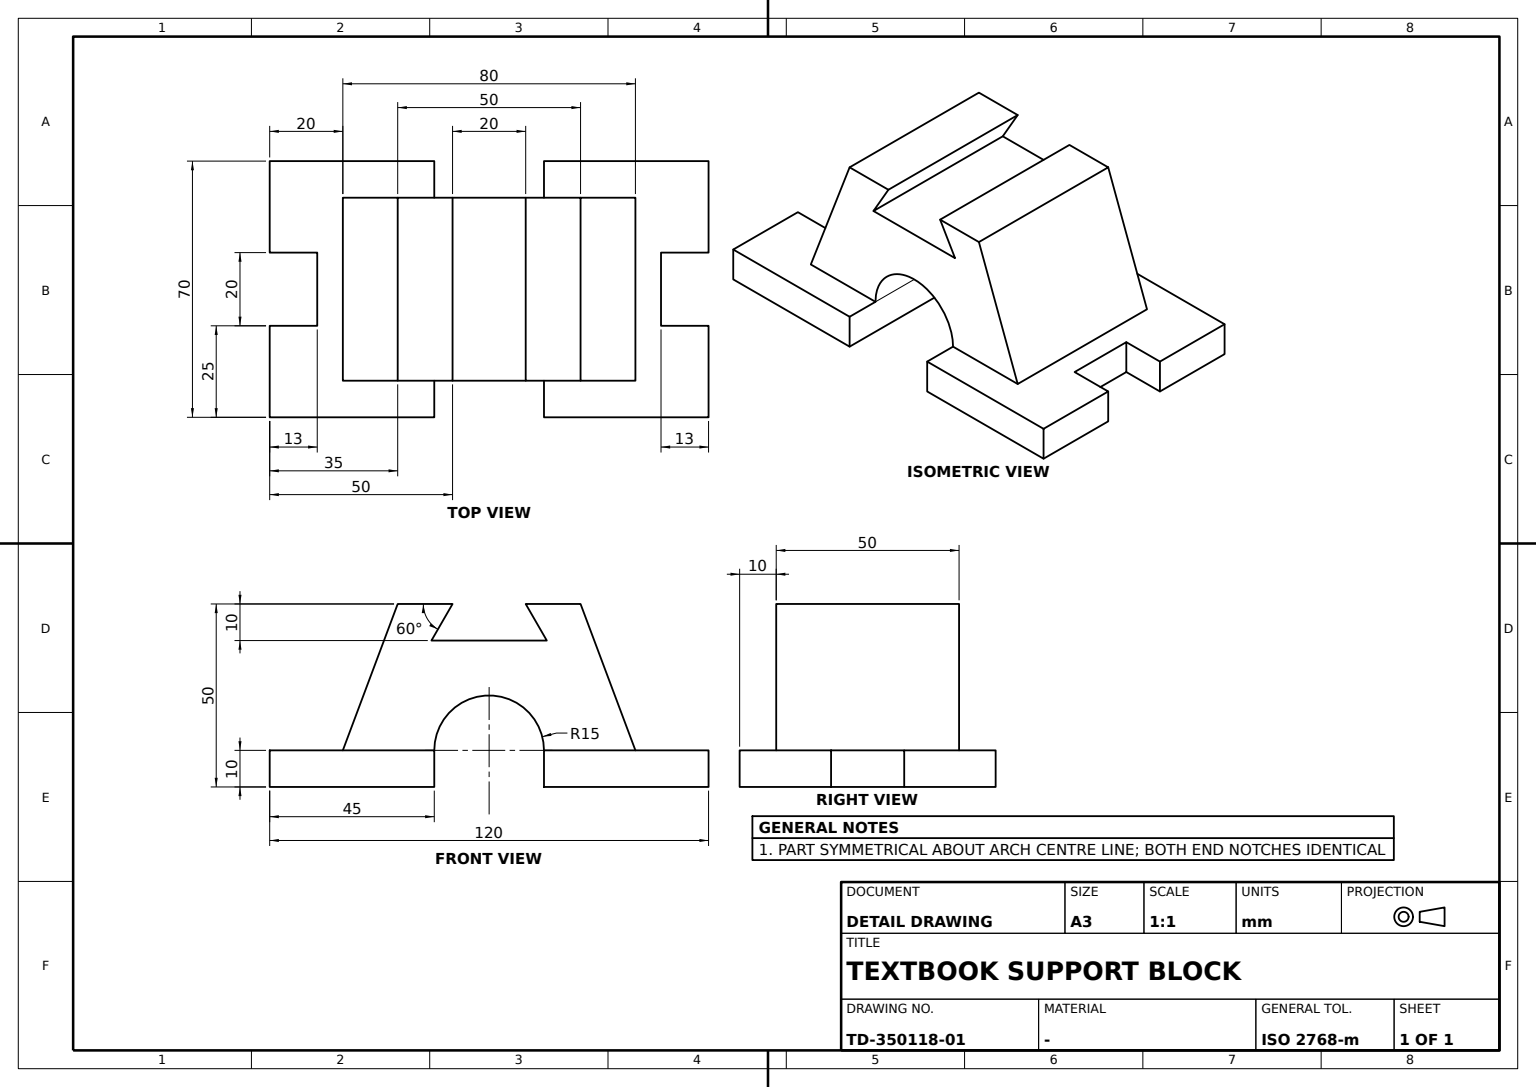
ISO-10303-21;
HEADER;
FILE_DESCRIPTION((''),'2;1');
FILE_NAME('','',(''),(''),'','','');
FILE_SCHEMA(('AUTOMOTIVE_DESIGN'));
ENDSEC;
DATA;
#1=APPLICATION_CONTEXT('');
#2=PRODUCT_CONTEXT('',#1,'mechanical');
#3=PRODUCT('','','',(#2));
#4=PRODUCT_DEFINITION_FORMATION('','',#3);
#5=PRODUCT_DEFINITION_CONTEXT('',#1,'design');
#6=PRODUCT_DEFINITION('','',#4,#5);
#7=PRODUCT_DEFINITION_SHAPE('','',#6);
#8=(LENGTH_UNIT()NAMED_UNIT(*)SI_UNIT(.MILLI.,.METRE.));
#9=(NAMED_UNIT(*)PLANE_ANGLE_UNIT()SI_UNIT($,.RADIAN.));
#10=(NAMED_UNIT(*)SI_UNIT($,.STERADIAN.)SOLID_ANGLE_UNIT());
#11=UNCERTAINTY_MEASURE_WITH_UNIT(LENGTH_MEASURE(1.E-05),#8,'distance_accuracy_value','');
#12=(GEOMETRIC_REPRESENTATION_CONTEXT(3)GLOBAL_UNCERTAINTY_ASSIGNED_CONTEXT((#11))GLOBAL_UNIT_ASSIGNED_CONTEXT((#8,#9,#10))REPRESENTATION_CONTEXT('',''));
#13=CARTESIAN_POINT('',(40.,25.,10.));
#14=VERTEX_POINT('',#13);
#15=CARTESIAN_POINT('',(15.,25.,10.));
#16=VERTEX_POINT('',#15);
#17=CARTESIAN_POINT('',(27.5,25.,10.));
#18=DIRECTION('',(-1.,0.,0.));
#19=VECTOR('',#18,1000.);
#20=LINE('',#17,#19);
#21=EDGE_CURVE('',#14,#16,#20,.T.);
#22=ORIENTED_EDGE('',*,*,#21,.F.);
#23=CARTESIAN_POINT('',(40.,-25.,10.));
#24=VERTEX_POINT('',#23);
#25=CARTESIAN_POINT('',(40.,0.,10.));
#26=DIRECTION('',(0.,1.,0.));
#27=VECTOR('',#26,1000.);
#28=LINE('',#25,#27);
#29=EDGE_CURVE('',#24,#14,#28,.T.);
#30=ORIENTED_EDGE('',*,*,#29,.F.);
#31=CARTESIAN_POINT('',(15.,-25.,10.));
#32=VERTEX_POINT('',#31);
#33=CARTESIAN_POINT('',(27.5,-25.,10.));
#34=LINE('',#33,#19);
#35=EDGE_CURVE('',#24,#32,#34,.T.);
#36=ORIENTED_EDGE('',*,*,#35,.T.);
#37=CARTESIAN_POINT('',(15.,-35.,10.));
#38=VERTEX_POINT('',#37);
#39=CARTESIAN_POINT('',(15.,-30.,10.));
#40=LINE('',#39,#27);
#41=EDGE_CURVE('',#38,#32,#40,.T.);
#42=ORIENTED_EDGE('',*,*,#41,.F.);
#43=CARTESIAN_POINT('',(60.,-35.,10.));
#44=VERTEX_POINT('',#43);
#45=CARTESIAN_POINT('',(37.5,-35.,10.));
#46=DIRECTION('',(1.,0.,0.));
#47=VECTOR('',#46,1000.);
#48=LINE('',#45,#47);
#49=EDGE_CURVE('',#38,#44,#48,.T.);
#50=ORIENTED_EDGE('',*,*,#49,.T.);
#51=CARTESIAN_POINT('',(60.,-10.,10.));
#52=VERTEX_POINT('',#51);
#53=CARTESIAN_POINT('',(60.,-22.5,10.));
#54=LINE('',#53,#27);
#55=EDGE_CURVE('',#44,#52,#54,.T.);
#56=ORIENTED_EDGE('',*,*,#55,.T.);
#57=CARTESIAN_POINT('',(47.,-10.,10.));
#58=VERTEX_POINT('',#57);
#59=CARTESIAN_POINT('',(53.5,-10.,10.));
#60=LINE('',#59,#47);
#61=EDGE_CURVE('',#58,#52,#60,.T.);
#62=ORIENTED_EDGE('',*,*,#61,.F.);
#63=CARTESIAN_POINT('',(47.,10.,10.));
#64=VERTEX_POINT('',#63);
#65=CARTESIAN_POINT('',(47.,0.,10.));
#66=DIRECTION('',(0.,-1.,0.));
#67=VECTOR('',#66,1000.);
#68=LINE('',#65,#67);
#69=EDGE_CURVE('',#64,#58,#68,.T.);
#70=ORIENTED_EDGE('',*,*,#69,.F.);
#71=CARTESIAN_POINT('',(60.,10.,10.));
#72=VERTEX_POINT('',#71);
#73=CARTESIAN_POINT('',(53.5,10.,10.));
#74=LINE('',#73,#19);
#75=EDGE_CURVE('',#72,#64,#74,.T.);
#76=ORIENTED_EDGE('',*,*,#75,.F.);
#77=CARTESIAN_POINT('',(60.,35.,10.));
#78=VERTEX_POINT('',#77);
#79=CARTESIAN_POINT('',(60.,22.5,10.));
#80=LINE('',#79,#27);
#81=EDGE_CURVE('',#72,#78,#80,.T.);
#82=ORIENTED_EDGE('',*,*,#81,.T.);
#83=CARTESIAN_POINT('',(15.,35.,10.));
#84=VERTEX_POINT('',#83);
#85=CARTESIAN_POINT('',(37.5,35.,10.));
#86=LINE('',#85,#19);
#87=EDGE_CURVE('',#78,#84,#86,.T.);
#88=ORIENTED_EDGE('',*,*,#87,.T.);
#89=CARTESIAN_POINT('',(15.,30.,10.));
#90=LINE('',#89,#27);
#91=EDGE_CURVE('',#16,#84,#90,.T.);
#92=ORIENTED_EDGE('',*,*,#91,.F.);
#93=EDGE_LOOP('',(#22,#30,#36,#42,#50,#56,#62,#70,#76,#82,#88,#92));
#94=FACE_OUTER_BOUND('',#93,.T.);
#95=CARTESIAN_POINT('',(0.,0.,10.));
#96=DIRECTION('',(0.,0.,1.));
#97=AXIS2_PLACEMENT_3D('',#95,#96,#46);
#98=PLANE('',#97);
#99=ADVANCED_FACE('',(#94),#98,.T.);
#100=CARTESIAN_POINT('',(25.,25.,50.));
#101=VERTEX_POINT('',#100);
#102=CARTESIAN_POINT('',(32.5,25.,30.));
#103=DIRECTION('',(0.351123442,0.,-0.936329178));
#104=VECTOR('',#103,1000.);
#105=LINE('',#102,#104);
#106=EDGE_CURVE('',#101,#14,#105,.T.);
#107=ORIENTED_EDGE('',*,*,#106,.T.);
#108=ORIENTED_EDGE('',*,*,#21,.T.);
#109=CARTESIAN_POINT('',(-15.,25.,10.));
#110=VERTEX_POINT('',#109);
#111=CARTESIAN_POINT('',(0.,25.,10.));
#112=AXIS2_PLACEMENT_3D('',#111,#26,#18);
#113=CIRCLE('',#112,15.);
#114=EDGE_CURVE('',#110,#16,#113,.T.);
#115=ORIENTED_EDGE('',*,*,#114,.F.);
#116=CARTESIAN_POINT('',(-40.,25.,10.));
#117=VERTEX_POINT('',#116);
#118=CARTESIAN_POINT('',(-27.5,25.,10.));
#119=LINE('',#118,#19);
#120=EDGE_CURVE('',#110,#117,#119,.T.);
#121=ORIENTED_EDGE('',*,*,#120,.T.);
#122=CARTESIAN_POINT('',(-25.,25.,50.));
#123=VERTEX_POINT('',#122);
#124=CARTESIAN_POINT('',(-32.5,25.,30.));
#125=DIRECTION('',(0.351123442,0.,0.936329178));
#126=VECTOR('',#125,1000.);
#127=LINE('',#124,#126);
#128=EDGE_CURVE('',#117,#123,#127,.T.);
#129=ORIENTED_EDGE('',*,*,#128,.T.);
#130=CARTESIAN_POINT('',(-10.,25.,50.));
#131=VERTEX_POINT('',#130);
#132=CARTESIAN_POINT('',(-17.5,25.,50.));
#133=LINE('',#132,#47);
#134=EDGE_CURVE('',#123,#131,#133,.T.);
#135=ORIENTED_EDGE('',*,*,#134,.T.);
#136=CARTESIAN_POINT('',(-15.773503,25.,40.));
#137=VERTEX_POINT('',#136);
#138=CARTESIAN_POINT('',(-12.886751,25.,45.));
#139=DIRECTION('',(-0.5,0.,-0.866025404));
#140=VECTOR('',#139,1000.);
#141=LINE('',#138,#140);
#142=EDGE_CURVE('',#131,#137,#141,.T.);
#143=ORIENTED_EDGE('',*,*,#142,.T.);
#144=CARTESIAN_POINT('',(15.773503,25.,40.));
#145=VERTEX_POINT('',#144);
#146=CARTESIAN_POINT('',(0.,25.,40.));
#147=LINE('',#146,#47);
#148=EDGE_CURVE('',#137,#145,#147,.T.);
#149=ORIENTED_EDGE('',*,*,#148,.T.);
#150=CARTESIAN_POINT('',(10.,25.,50.));
#151=VERTEX_POINT('',#150);
#152=CARTESIAN_POINT('',(12.886751,25.,45.));
#153=DIRECTION('',(0.5,0.,-0.866025404));
#154=VECTOR('',#153,1000.);
#155=LINE('',#152,#154);
#156=EDGE_CURVE('',#151,#145,#155,.T.);
#157=ORIENTED_EDGE('',*,*,#156,.F.);
#158=CARTESIAN_POINT('',(17.5,25.,50.));
#159=LINE('',#158,#47);
#160=EDGE_CURVE('',#151,#101,#159,.T.);
#161=ORIENTED_EDGE('',*,*,#160,.T.);
#162=EDGE_LOOP('',(#107,#108,#115,#121,#129,#135,#143,#149,#157,#161));
#163=FACE_OUTER_BOUND('',#162,.T.);
#164=CARTESIAN_POINT('',(0.,25.,0.));
#165=AXIS2_PLACEMENT_3D('',#164,#26,#18);
#166=PLANE('',#165);
#167=ADVANCED_FACE('',(#163),#166,.T.);
#168=CARTESIAN_POINT('',(-60.,-10.,0.));
#169=VERTEX_POINT('',#168);
#170=CARTESIAN_POINT('',(-47.,-10.,0.));
#171=VERTEX_POINT('',#170);
#172=CARTESIAN_POINT('',(-53.5,-10.,0.));
#173=LINE('',#172,#47);
#174=EDGE_CURVE('',#169,#171,#173,.T.);
#175=ORIENTED_EDGE('',*,*,#174,.T.);
#176=CARTESIAN_POINT('',(-47.,10.,0.));
#177=VERTEX_POINT('',#176);
#178=CARTESIAN_POINT('',(-47.,0.,0.));
#179=LINE('',#178,#27);
#180=EDGE_CURVE('',#171,#177,#179,.T.);
#181=ORIENTED_EDGE('',*,*,#180,.T.);
#182=CARTESIAN_POINT('',(-60.,10.,0.));
#183=VERTEX_POINT('',#182);
#184=CARTESIAN_POINT('',(-53.5,10.,0.));
#185=LINE('',#184,#47);
#186=EDGE_CURVE('',#183,#177,#185,.T.);
#187=ORIENTED_EDGE('',*,*,#186,.F.);
#188=CARTESIAN_POINT('',(-60.,35.,0.));
#189=VERTEX_POINT('',#188);
#190=CARTESIAN_POINT('',(-60.,22.5,0.));
#191=LINE('',#190,#67);
#192=EDGE_CURVE('',#189,#183,#191,.T.);
#193=ORIENTED_EDGE('',*,*,#192,.F.);
#194=CARTESIAN_POINT('',(-15.,35.,0.));
#195=VERTEX_POINT('',#194);
#196=CARTESIAN_POINT('',(-37.5,35.,0.));
#197=LINE('',#196,#19);
#198=EDGE_CURVE('',#195,#189,#197,.T.);
#199=ORIENTED_EDGE('',*,*,#198,.F.);
#200=CARTESIAN_POINT('',(-15.,-35.,0.));
#201=VERTEX_POINT('',#200);
#202=CARTESIAN_POINT('',(-15.,0.,0.));
#203=LINE('',#202,#27);
#204=EDGE_CURVE('',#201,#195,#203,.T.);
#205=ORIENTED_EDGE('',*,*,#204,.F.);
#206=CARTESIAN_POINT('',(-60.,-35.,0.));
#207=VERTEX_POINT('',#206);
#208=CARTESIAN_POINT('',(-37.5,-35.,0.));
#209=LINE('',#208,#47);
#210=EDGE_CURVE('',#207,#201,#209,.T.);
#211=ORIENTED_EDGE('',*,*,#210,.F.);
#212=CARTESIAN_POINT('',(-60.,-22.5,0.));
#213=LINE('',#212,#67);
#214=EDGE_CURVE('',#169,#207,#213,.T.);
#215=ORIENTED_EDGE('',*,*,#214,.F.);
#216=EDGE_LOOP('',(#175,#181,#187,#193,#199,#205,#211,#215));
#217=FACE_OUTER_BOUND('',#216,.T.);
#218=CARTESIAN_POINT('',(0.,0.,0.));
#219=AXIS2_PLACEMENT_3D('',#218,#96,#46);
#220=PLANE('',#219);
#221=ADVANCED_FACE('',(#217),#220,.F.);
#222=CARTESIAN_POINT('',(47.,10.,0.));
#223=VERTEX_POINT('',#222);
#224=CARTESIAN_POINT('',(47.,10.,5.));
#225=DIRECTION('',(0.,0.,-1.));
#226=VECTOR('',#225,1000.);
#227=LINE('',#224,#226);
#228=EDGE_CURVE('',#64,#223,#227,.T.);
#229=ORIENTED_EDGE('',*,*,#228,.F.);
#230=ORIENTED_EDGE('',*,*,#69,.T.);
#231=CARTESIAN_POINT('',(47.,-10.,0.));
#232=VERTEX_POINT('',#231);
#233=CARTESIAN_POINT('',(47.,-10.,5.));
#234=LINE('',#233,#226);
#235=EDGE_CURVE('',#58,#232,#234,.T.);
#236=ORIENTED_EDGE('',*,*,#235,.T.);
#237=CARTESIAN_POINT('',(47.,0.,0.));
#238=LINE('',#237,#27);
#239=EDGE_CURVE('',#232,#223,#238,.T.);
#240=ORIENTED_EDGE('',*,*,#239,.T.);
#241=EDGE_LOOP('',(#229,#230,#236,#240));
#242=FACE_OUTER_BOUND('',#241,.T.);
#243=AXIS2_PLACEMENT_3D('',#57,#18,#26);
#244=PLANE('',#243);
#245=ADVANCED_FACE('',(#242),#244,.F.);
#246=CARTESIAN_POINT('',(60.,-35.,0.));
#247=VERTEX_POINT('',#246);
#248=CARTESIAN_POINT('',(60.,-35.,5.));
#249=VECTOR('',#96,1000.);
#250=LINE('',#248,#249);
#251=EDGE_CURVE('',#247,#44,#250,.T.);
#252=ORIENTED_EDGE('',*,*,#251,.T.);
#253=ORIENTED_EDGE('',*,*,#49,.F.);
#254=CARTESIAN_POINT('',(15.,-35.,0.));
#255=VERTEX_POINT('',#254);
#256=CARTESIAN_POINT('',(15.,-35.,5.));
#257=LINE('',#256,#249);
#258=EDGE_CURVE('',#255,#38,#257,.T.);
#259=ORIENTED_EDGE('',*,*,#258,.F.);
#260=CARTESIAN_POINT('',(37.5,-35.,0.));
#261=LINE('',#260,#47);
#262=EDGE_CURVE('',#255,#247,#261,.T.);
#263=ORIENTED_EDGE('',*,*,#262,.T.);
#264=EDGE_LOOP('',(#252,#253,#259,#263));
#265=FACE_OUTER_BOUND('',#264,.T.);
#266=AXIS2_PLACEMENT_3D('',#246,#26,#18);
#267=PLANE('',#266);
#268=ADVANCED_FACE('',(#265),#267,.F.);
#269=CARTESIAN_POINT('',(60.,10.,0.));
#270=VERTEX_POINT('',#269);
#271=CARTESIAN_POINT('',(60.,10.,5.));
#272=LINE('',#271,#226);
#273=EDGE_CURVE('',#72,#270,#272,.T.);
#274=ORIENTED_EDGE('',*,*,#273,.F.);
#275=ORIENTED_EDGE('',*,*,#75,.T.);
#276=ORIENTED_EDGE('',*,*,#228,.T.);
#277=CARTESIAN_POINT('',(53.5,10.,0.));
#278=LINE('',#277,#19);
#279=EDGE_CURVE('',#270,#223,#278,.T.);
#280=ORIENTED_EDGE('',*,*,#279,.F.);
#281=EDGE_LOOP('',(#274,#275,#276,#280));
#282=FACE_OUTER_BOUND('',#281,.T.);
#283=AXIS2_PLACEMENT_3D('',#63,#26,#46);
#284=PLANE('',#283);
#285=ADVANCED_FACE('',(#282),#284,.F.);
#286=CARTESIAN_POINT('',(-15.,-35.,10.));
#287=VERTEX_POINT('',#286);
#288=CARTESIAN_POINT('',(-15.,-35.,5.));
#289=LINE('',#288,#226);
#290=EDGE_CURVE('',#287,#201,#289,.T.);
#291=ORIENTED_EDGE('',*,*,#290,.F.);
#292=CARTESIAN_POINT('',(-60.,-35.,10.));
#293=VERTEX_POINT('',#292);
#294=CARTESIAN_POINT('',(-37.5,-35.,10.));
#295=LINE('',#294,#47);
#296=EDGE_CURVE('',#293,#287,#295,.T.);
#297=ORIENTED_EDGE('',*,*,#296,.F.);
#298=CARTESIAN_POINT('',(-60.,-35.,5.));
#299=LINE('',#298,#249);
#300=EDGE_CURVE('',#207,#293,#299,.T.);
#301=ORIENTED_EDGE('',*,*,#300,.F.);
#302=ORIENTED_EDGE('',*,*,#210,.T.);
#303=EDGE_LOOP('',(#291,#297,#301,#302));
#304=FACE_OUTER_BOUND('',#303,.T.);
#305=ADVANCED_FACE('',(#304),#267,.F.);
#306=CARTESIAN_POINT('',(-40.,-25.,10.));
#307=VERTEX_POINT('',#306);
#308=CARTESIAN_POINT('',(-40.,0.,10.));
#309=LINE('',#308,#27);
#310=EDGE_CURVE('',#307,#117,#309,.T.);
#311=ORIENTED_EDGE('',*,*,#310,.F.);
#312=CARTESIAN_POINT('',(-25.,-25.,50.));
#313=VERTEX_POINT('',#312);
#314=CARTESIAN_POINT('',(-32.5,-25.,30.));
#315=LINE('',#314,#126);
#316=EDGE_CURVE('',#307,#313,#315,.T.);
#317=ORIENTED_EDGE('',*,*,#316,.T.);
#318=CARTESIAN_POINT('',(-25.,0.,50.));
#319=LINE('',#318,#27);
#320=EDGE_CURVE('',#313,#123,#319,.T.);
#321=ORIENTED_EDGE('',*,*,#320,.T.);
#322=ORIENTED_EDGE('',*,*,#128,.F.);
#323=EDGE_LOOP('',(#311,#317,#321,#322));
#324=FACE_OUTER_BOUND('',#323,.T.);
#325=DIRECTION('',(0.936329178,0.,-0.351123442));
#326=DIRECTION('',(-0.351123442,0.,-0.936329178));
#327=AXIS2_PLACEMENT_3D('',#318,#325,#326);
#328=PLANE('',#327);
#329=ADVANCED_FACE('',(#324),#328,.F.);
#330=CARTESIAN_POINT('',(-47.,10.,10.));
#331=VERTEX_POINT('',#330);
#332=CARTESIAN_POINT('',(-47.,10.,5.));
#333=LINE('',#332,#226);
#334=EDGE_CURVE('',#331,#177,#333,.T.);
#335=ORIENTED_EDGE('',*,*,#334,.T.);
#336=ORIENTED_EDGE('',*,*,#180,.F.);
#337=CARTESIAN_POINT('',(-47.,-10.,10.));
#338=VERTEX_POINT('',#337);
#339=CARTESIAN_POINT('',(-47.,-10.,5.));
#340=LINE('',#339,#226);
#341=EDGE_CURVE('',#338,#171,#340,.T.);
#342=ORIENTED_EDGE('',*,*,#341,.F.);
#343=CARTESIAN_POINT('',(-47.,0.,10.));
#344=LINE('',#343,#27);
#345=EDGE_CURVE('',#338,#331,#344,.T.);
#346=ORIENTED_EDGE('',*,*,#345,.T.);
#347=EDGE_LOOP('',(#335,#336,#342,#346));
#348=FACE_OUTER_BOUND('',#347,.T.);
#349=AXIS2_PLACEMENT_3D('',#337,#18,#26);
#350=PLANE('',#349);
#351=ADVANCED_FACE('',(#348),#350,.T.);
#352=ORIENTED_EDGE('',*,*,#262,.F.);
#353=CARTESIAN_POINT('',(15.,35.,0.));
#354=VERTEX_POINT('',#353);
#355=CARTESIAN_POINT('',(15.,0.,0.));
#356=LINE('',#355,#27);
#357=EDGE_CURVE('',#255,#354,#356,.T.);
#358=ORIENTED_EDGE('',*,*,#357,.T.);
#359=CARTESIAN_POINT('',(60.,35.,0.));
#360=VERTEX_POINT('',#359);
#361=CARTESIAN_POINT('',(37.5,35.,0.));
#362=LINE('',#361,#19);
#363=EDGE_CURVE('',#360,#354,#362,.T.);
#364=ORIENTED_EDGE('',*,*,#363,.F.);
#365=CARTESIAN_POINT('',(60.,22.5,0.));
#366=LINE('',#365,#27);
#367=EDGE_CURVE('',#270,#360,#366,.T.);
#368=ORIENTED_EDGE('',*,*,#367,.F.);
#369=ORIENTED_EDGE('',*,*,#279,.T.);
#370=ORIENTED_EDGE('',*,*,#239,.F.);
#371=CARTESIAN_POINT('',(60.,-10.,0.));
#372=VERTEX_POINT('',#371);
#373=CARTESIAN_POINT('',(53.5,-10.,0.));
#374=LINE('',#373,#19);
#375=EDGE_CURVE('',#372,#232,#374,.T.);
#376=ORIENTED_EDGE('',*,*,#375,.F.);
#377=CARTESIAN_POINT('',(60.,-22.5,0.));
#378=LINE('',#377,#27);
#379=EDGE_CURVE('',#247,#372,#378,.T.);
#380=ORIENTED_EDGE('',*,*,#379,.F.);
#381=EDGE_LOOP('',(#352,#358,#364,#368,#369,#370,#376,#380));
#382=FACE_OUTER_BOUND('',#381,.T.);
#383=ADVANCED_FACE('',(#382),#220,.F.);
#384=ORIENTED_EDGE('',*,*,#148,.F.);
#385=CARTESIAN_POINT('',(-15.773503,-25.,40.));
#386=VERTEX_POINT('',#385);
#387=CARTESIAN_POINT('',(-15.773503,0.,40.));
#388=LINE('',#387,#27);
#389=EDGE_CURVE('',#386,#137,#388,.T.);
#390=ORIENTED_EDGE('',*,*,#389,.F.);
#391=CARTESIAN_POINT('',(15.773503,-25.,40.));
#392=VERTEX_POINT('',#391);
#393=CARTESIAN_POINT('',(0.,-25.,40.));
#394=LINE('',#393,#47);
#395=EDGE_CURVE('',#386,#392,#394,.T.);
#396=ORIENTED_EDGE('',*,*,#395,.T.);
#397=CARTESIAN_POINT('',(15.773503,0.,40.));
#398=LINE('',#397,#27);
#399=EDGE_CURVE('',#392,#145,#398,.T.);
#400=ORIENTED_EDGE('',*,*,#399,.T.);
#401=EDGE_LOOP('',(#384,#390,#396,#400));
#402=FACE_OUTER_BOUND('',#401,.T.);
#403=AXIS2_PLACEMENT_3D('',#385,#96,#46);
#404=PLANE('',#403);
#405=ADVANCED_FACE('',(#402),#404,.T.);
#406=ORIENTED_EDGE('',*,*,#198,.T.);
#407=CARTESIAN_POINT('',(-60.,35.,10.));
#408=VERTEX_POINT('',#407);
#409=CARTESIAN_POINT('',(-60.,35.,5.));
#410=LINE('',#409,#249);
#411=EDGE_CURVE('',#189,#408,#410,.T.);
#412=ORIENTED_EDGE('',*,*,#411,.T.);
#413=CARTESIAN_POINT('',(-15.,35.,10.));
#414=VERTEX_POINT('',#413);
#415=CARTESIAN_POINT('',(-37.5,35.,10.));
#416=LINE('',#415,#19);
#417=EDGE_CURVE('',#414,#408,#416,.T.);
#418=ORIENTED_EDGE('',*,*,#417,.F.);
#419=CARTESIAN_POINT('',(-15.,35.,5.));
#420=LINE('',#419,#249);
#421=EDGE_CURVE('',#195,#414,#420,.T.);
#422=ORIENTED_EDGE('',*,*,#421,.F.);
#423=EDGE_LOOP('',(#406,#412,#418,#422));
#424=FACE_OUTER_BOUND('',#423,.T.);
#425=AXIS2_PLACEMENT_3D('',#188,#66,#46);
#426=PLANE('',#425);
#427=ADVANCED_FACE('',(#424),#426,.F.);
#428=ORIENTED_EDGE('',*,*,#258,.T.);
#429=ORIENTED_EDGE('',*,*,#41,.T.);
#430=CARTESIAN_POINT('',(15.,0.,10.));
#431=LINE('',#430,#27);
#432=EDGE_CURVE('',#32,#16,#431,.T.);
#433=ORIENTED_EDGE('',*,*,#432,.T.);
#434=ORIENTED_EDGE('',*,*,#91,.T.);
#435=CARTESIAN_POINT('',(15.,35.,5.));
#436=LINE('',#435,#249);
#437=EDGE_CURVE('',#354,#84,#436,.T.);
#438=ORIENTED_EDGE('',*,*,#437,.F.);
#439=ORIENTED_EDGE('',*,*,#357,.F.);
#440=EDGE_LOOP('',(#428,#429,#433,#434,#438,#439));
#441=FACE_OUTER_BOUND('',#440,.T.);
#442=AXIS2_PLACEMENT_3D('',#254,#18,#96);
#443=PLANE('',#442);
#444=ADVANCED_FACE('',(#441),#443,.T.);
#445=ORIENTED_EDGE('',*,*,#290,.T.);
#446=ORIENTED_EDGE('',*,*,#204,.T.);
#447=ORIENTED_EDGE('',*,*,#421,.T.);
#448=CARTESIAN_POINT('',(-15.,30.,10.));
#449=LINE('',#448,#27);
#450=EDGE_CURVE('',#110,#414,#449,.T.);
#451=ORIENTED_EDGE('',*,*,#450,.F.);
#452=CARTESIAN_POINT('',(-15.,-25.,10.));
#453=VERTEX_POINT('',#452);
#454=CARTESIAN_POINT('',(-15.,0.66,10.));
#455=LINE('',#454,#27);
#456=EDGE_CURVE('',#453,#110,#455,.T.);
#457=ORIENTED_EDGE('',*,*,#456,.F.);
#458=CARTESIAN_POINT('',(-15.,-30.,10.));
#459=LINE('',#458,#27);
#460=EDGE_CURVE('',#287,#453,#459,.T.);
#461=ORIENTED_EDGE('',*,*,#460,.F.);
#462=EDGE_LOOP('',(#445,#446,#447,#451,#457,#461));
#463=FACE_OUTER_BOUND('',#462,.T.);
#464=AXIS2_PLACEMENT_3D('',#200,#18,#96);
#465=PLANE('',#464);
#466=ADVANCED_FACE('',(#463),#465,.F.);
#467=CARTESIAN_POINT('',(-60.,-10.,10.));
#468=VERTEX_POINT('',#467);
#469=CARTESIAN_POINT('',(-53.5,-10.,10.));
#470=LINE('',#469,#47);
#471=EDGE_CURVE('',#468,#338,#470,.T.);
#472=ORIENTED_EDGE('',*,*,#471,.T.);
#473=ORIENTED_EDGE('',*,*,#341,.T.);
#474=ORIENTED_EDGE('',*,*,#174,.F.);
#475=CARTESIAN_POINT('',(-60.,-10.,5.));
#476=LINE('',#475,#226);
#477=EDGE_CURVE('',#468,#169,#476,.T.);
#478=ORIENTED_EDGE('',*,*,#477,.F.);
#479=EDGE_LOOP('',(#472,#473,#474,#478));
#480=FACE_OUTER_BOUND('',#479,.T.);
#481=AXIS2_PLACEMENT_3D('',#51,#66,#18);
#482=PLANE('',#481);
#483=ADVANCED_FACE('',(#480),#482,.F.);
#484=ORIENTED_EDGE('',*,*,#477,.T.);
#485=ORIENTED_EDGE('',*,*,#214,.T.);
#486=ORIENTED_EDGE('',*,*,#300,.T.);
#487=CARTESIAN_POINT('',(-60.,-22.5,10.));
#488=LINE('',#487,#67);
#489=EDGE_CURVE('',#468,#293,#488,.T.);
#490=ORIENTED_EDGE('',*,*,#489,.F.);
#491=EDGE_LOOP('',(#484,#485,#486,#490));
#492=FACE_OUTER_BOUND('',#491,.T.);
#493=AXIS2_PLACEMENT_3D('',#206,#46,#26);
#494=PLANE('',#493);
#495=ADVANCED_FACE('',(#492),#494,.F.);
#496=ORIENTED_EDGE('',*,*,#156,.T.);
#497=ORIENTED_EDGE('',*,*,#399,.F.);
#498=CARTESIAN_POINT('',(10.,-25.,50.));
#499=VERTEX_POINT('',#498);
#500=CARTESIAN_POINT('',(12.886751,-25.,45.));
#501=DIRECTION('',(-0.5,0.,0.866025404));
#502=VECTOR('',#501,1000.);
#503=LINE('',#500,#502);
#504=EDGE_CURVE('',#392,#499,#503,.T.);
#505=ORIENTED_EDGE('',*,*,#504,.T.);
#506=CARTESIAN_POINT('',(10.,0.,50.));
#507=LINE('',#506,#27);
#508=EDGE_CURVE('',#499,#151,#507,.T.);
#509=ORIENTED_EDGE('',*,*,#508,.T.);
#510=EDGE_LOOP('',(#496,#497,#505,#509));
#511=FACE_OUTER_BOUND('',#510,.T.);
#512=DIRECTION('',(0.866025404,0.,0.5));
#513=AXIS2_PLACEMENT_3D('',#498,#512,#153);
#514=PLANE('',#513);
#515=ADVANCED_FACE('',(#511),#514,.F.);
#516=CARTESIAN_POINT('',(0.,-25.,10.));
#517=AXIS2_PLACEMENT_3D('',#516,#26,#18);
#518=CIRCLE('',#517,15.);
#519=EDGE_CURVE('',#453,#32,#518,.T.);
#520=ORIENTED_EDGE('',*,*,#519,.F.);
#521=ORIENTED_EDGE('',*,*,#456,.T.);
#522=ORIENTED_EDGE('',*,*,#114,.T.);
#523=ORIENTED_EDGE('',*,*,#432,.F.);
#524=EDGE_LOOP('',(#520,#521,#522,#523));
#525=FACE_OUTER_BOUND('',#524,.T.);
#526=CARTESIAN_POINT('',(0.,0.66,10.));
#527=AXIS2_PLACEMENT_3D('',#526,#26,#46);
#528=CYLINDRICAL_SURFACE('',#527,15.);
#529=ADVANCED_FACE('',(#525),#528,.F.);
#530=ORIENTED_EDGE('',*,*,#367,.T.);
#531=CARTESIAN_POINT('',(60.,35.,5.));
#532=LINE('',#531,#249);
#533=EDGE_CURVE('',#360,#78,#532,.T.);
#534=ORIENTED_EDGE('',*,*,#533,.T.);
#535=ORIENTED_EDGE('',*,*,#81,.F.);
#536=ORIENTED_EDGE('',*,*,#273,.T.);
#537=EDGE_LOOP('',(#530,#534,#535,#536));
#538=FACE_OUTER_BOUND('',#537,.T.);
#539=AXIS2_PLACEMENT_3D('',#359,#18,#66);
#540=PLANE('',#539);
#541=ADVANCED_FACE('',(#538),#540,.F.);
#542=ORIENTED_EDGE('',*,*,#411,.F.);
#543=ORIENTED_EDGE('',*,*,#192,.T.);
#544=CARTESIAN_POINT('',(-60.,10.,10.));
#545=VERTEX_POINT('',#544);
#546=CARTESIAN_POINT('',(-60.,10.,5.));
#547=LINE('',#546,#226);
#548=EDGE_CURVE('',#545,#183,#547,.T.);
#549=ORIENTED_EDGE('',*,*,#548,.F.);
#550=CARTESIAN_POINT('',(-60.,22.5,10.));
#551=LINE('',#550,#67);
#552=EDGE_CURVE('',#408,#545,#551,.T.);
#553=ORIENTED_EDGE('',*,*,#552,.F.);
#554=EDGE_LOOP('',(#542,#543,#549,#553));
#555=FACE_OUTER_BOUND('',#554,.T.);
#556=ADVANCED_FACE('',(#555),#494,.F.);
#557=ORIENTED_EDGE('',*,*,#489,.T.);
#558=ORIENTED_EDGE('',*,*,#296,.T.);
#559=ORIENTED_EDGE('',*,*,#460,.T.);
#560=CARTESIAN_POINT('',(-27.5,-25.,10.));
#561=LINE('',#560,#19);
#562=EDGE_CURVE('',#453,#307,#561,.T.);
#563=ORIENTED_EDGE('',*,*,#562,.T.);
#564=ORIENTED_EDGE('',*,*,#310,.T.);
#565=ORIENTED_EDGE('',*,*,#120,.F.);
#566=ORIENTED_EDGE('',*,*,#450,.T.);
#567=ORIENTED_EDGE('',*,*,#417,.T.);
#568=ORIENTED_EDGE('',*,*,#552,.T.);
#569=CARTESIAN_POINT('',(-53.5,10.,10.));
#570=LINE('',#569,#19);
#571=EDGE_CURVE('',#331,#545,#570,.T.);
#572=ORIENTED_EDGE('',*,*,#571,.F.);
#573=ORIENTED_EDGE('',*,*,#345,.F.);
#574=ORIENTED_EDGE('',*,*,#471,.F.);
#575=EDGE_LOOP('',(#557,#558,#559,#563,#564,#565,#566,#567,#568,#572,#573,#574));
#576=FACE_OUTER_BOUND('',#575,.T.);
#577=ADVANCED_FACE('',(#576),#98,.T.);
#578=ORIENTED_EDGE('',*,*,#106,.F.);
#579=CARTESIAN_POINT('',(25.,-25.,50.));
#580=VERTEX_POINT('',#579);
#581=CARTESIAN_POINT('',(25.,0.,50.));
#582=LINE('',#581,#27);
#583=EDGE_CURVE('',#580,#101,#582,.T.);
#584=ORIENTED_EDGE('',*,*,#583,.F.);
#585=CARTESIAN_POINT('',(32.5,-25.,30.));
#586=LINE('',#585,#104);
#587=EDGE_CURVE('',#580,#24,#586,.T.);
#588=ORIENTED_EDGE('',*,*,#587,.T.);
#589=ORIENTED_EDGE('',*,*,#29,.T.);
#590=EDGE_LOOP('',(#578,#584,#588,#589));
#591=FACE_OUTER_BOUND('',#590,.T.);
#592=DIRECTION('',(0.936329178,0.,0.351123442));
#593=AXIS2_PLACEMENT_3D('',#581,#592,#103);
#594=PLANE('',#593);
#595=ADVANCED_FACE('',(#591),#594,.T.);
#596=ORIENTED_EDGE('',*,*,#395,.F.);
#597=CARTESIAN_POINT('',(-10.,-25.,50.));
#598=VERTEX_POINT('',#597);
#599=CARTESIAN_POINT('',(-12.886751,-25.,45.));
#600=LINE('',#599,#140);
#601=EDGE_CURVE('',#598,#386,#600,.T.);
#602=ORIENTED_EDGE('',*,*,#601,.F.);
#603=CARTESIAN_POINT('',(-17.5,-25.,50.));
#604=LINE('',#603,#47);
#605=EDGE_CURVE('',#313,#598,#604,.T.);
#606=ORIENTED_EDGE('',*,*,#605,.F.);
#607=ORIENTED_EDGE('',*,*,#316,.F.);
#608=ORIENTED_EDGE('',*,*,#562,.F.);
#609=ORIENTED_EDGE('',*,*,#519,.T.);
#610=ORIENTED_EDGE('',*,*,#35,.F.);
#611=ORIENTED_EDGE('',*,*,#587,.F.);
#612=CARTESIAN_POINT('',(17.5,-25.,50.));
#613=LINE('',#612,#47);
#614=EDGE_CURVE('',#499,#580,#613,.T.);
#615=ORIENTED_EDGE('',*,*,#614,.F.);
#616=ORIENTED_EDGE('',*,*,#504,.F.);
#617=EDGE_LOOP('',(#596,#602,#606,#607,#608,#609,#610,#611,#615,#616));
#618=FACE_OUTER_BOUND('',#617,.T.);
#619=CARTESIAN_POINT('',(0.,-25.,0.));
#620=AXIS2_PLACEMENT_3D('',#619,#26,#18);
#621=PLANE('',#620);
#622=ADVANCED_FACE('',(#618),#621,.F.);
#623=CARTESIAN_POINT('',(60.,-10.,5.));
#624=LINE('',#623,#226);
#625=EDGE_CURVE('',#52,#372,#624,.T.);
#626=ORIENTED_EDGE('',*,*,#625,.T.);
#627=ORIENTED_EDGE('',*,*,#375,.T.);
#628=ORIENTED_EDGE('',*,*,#235,.F.);
#629=ORIENTED_EDGE('',*,*,#61,.T.);
#630=EDGE_LOOP('',(#626,#627,#628,#629));
#631=FACE_OUTER_BOUND('',#630,.T.);
#632=ADVANCED_FACE('',(#631),#482,.F.);
#633=ORIENTED_EDGE('',*,*,#605,.T.);
#634=CARTESIAN_POINT('',(-10.,0.,50.));
#635=LINE('',#634,#27);
#636=EDGE_CURVE('',#598,#131,#635,.T.);
#637=ORIENTED_EDGE('',*,*,#636,.T.);
#638=ORIENTED_EDGE('',*,*,#134,.F.);
#639=ORIENTED_EDGE('',*,*,#320,.F.);
#640=EDGE_LOOP('',(#633,#637,#638,#639));
#641=FACE_OUTER_BOUND('',#640,.T.);
#642=AXIS2_PLACEMENT_3D('',#581,#225,#18);
#643=PLANE('',#642);
#644=ADVANCED_FACE('',(#641),#643,.F.);
#645=ORIENTED_EDGE('',*,*,#363,.T.);
#646=ORIENTED_EDGE('',*,*,#437,.T.);
#647=ORIENTED_EDGE('',*,*,#87,.F.);
#648=ORIENTED_EDGE('',*,*,#533,.F.);
#649=EDGE_LOOP('',(#645,#646,#647,#648));
#650=FACE_OUTER_BOUND('',#649,.T.);
#651=ADVANCED_FACE('',(#650),#426,.F.);
#652=ORIENTED_EDGE('',*,*,#186,.T.);
#653=ORIENTED_EDGE('',*,*,#334,.F.);
#654=ORIENTED_EDGE('',*,*,#571,.T.);
#655=ORIENTED_EDGE('',*,*,#548,.T.);
#656=EDGE_LOOP('',(#652,#653,#654,#655));
#657=FACE_OUTER_BOUND('',#656,.T.);
#658=ADVANCED_FACE('',(#657),#284,.F.);
#659=ORIENTED_EDGE('',*,*,#636,.F.);
#660=ORIENTED_EDGE('',*,*,#601,.T.);
#661=ORIENTED_EDGE('',*,*,#389,.T.);
#662=ORIENTED_EDGE('',*,*,#142,.F.);
#663=EDGE_LOOP('',(#659,#660,#661,#662));
#664=FACE_OUTER_BOUND('',#663,.T.);
#665=DIRECTION('',(0.866025404,0.,-0.5));
#666=AXIS2_PLACEMENT_3D('',#597,#665,#139);
#667=PLANE('',#666);
#668=ADVANCED_FACE('',(#664),#667,.T.);
#669=ORIENTED_EDGE('',*,*,#583,.T.);
#670=ORIENTED_EDGE('',*,*,#160,.F.);
#671=ORIENTED_EDGE('',*,*,#508,.F.);
#672=ORIENTED_EDGE('',*,*,#614,.T.);
#673=EDGE_LOOP('',(#669,#670,#671,#672));
#674=FACE_OUTER_BOUND('',#673,.T.);
#675=ADVANCED_FACE('',(#674),#643,.F.);
#676=ORIENTED_EDGE('',*,*,#625,.F.);
#677=ORIENTED_EDGE('',*,*,#55,.F.);
#678=ORIENTED_EDGE('',*,*,#251,.F.);
#679=ORIENTED_EDGE('',*,*,#379,.T.);
#680=EDGE_LOOP('',(#676,#677,#678,#679));
#681=FACE_OUTER_BOUND('',#680,.T.);
#682=ADVANCED_FACE('',(#681),#540,.F.);
#683=CLOSED_SHELL('',(#99,#167,#221,#245,#268,#285,#305,#329,#351,#383,#405,#427,#444,#466,#483,#495,#515,#529,#541,#556,#577,#595,#622,#632,#644,#651,#658,#668,#675,#682));
#684=MANIFOLD_SOLID_BREP('',#683);
#685=ADVANCED_BREP_SHAPE_REPRESENTATION('',(#684),#12);
#686=SHAPE_DEFINITION_REPRESENTATION(#7,#685);
ENDSEC;
END-ISO-10303-21;
